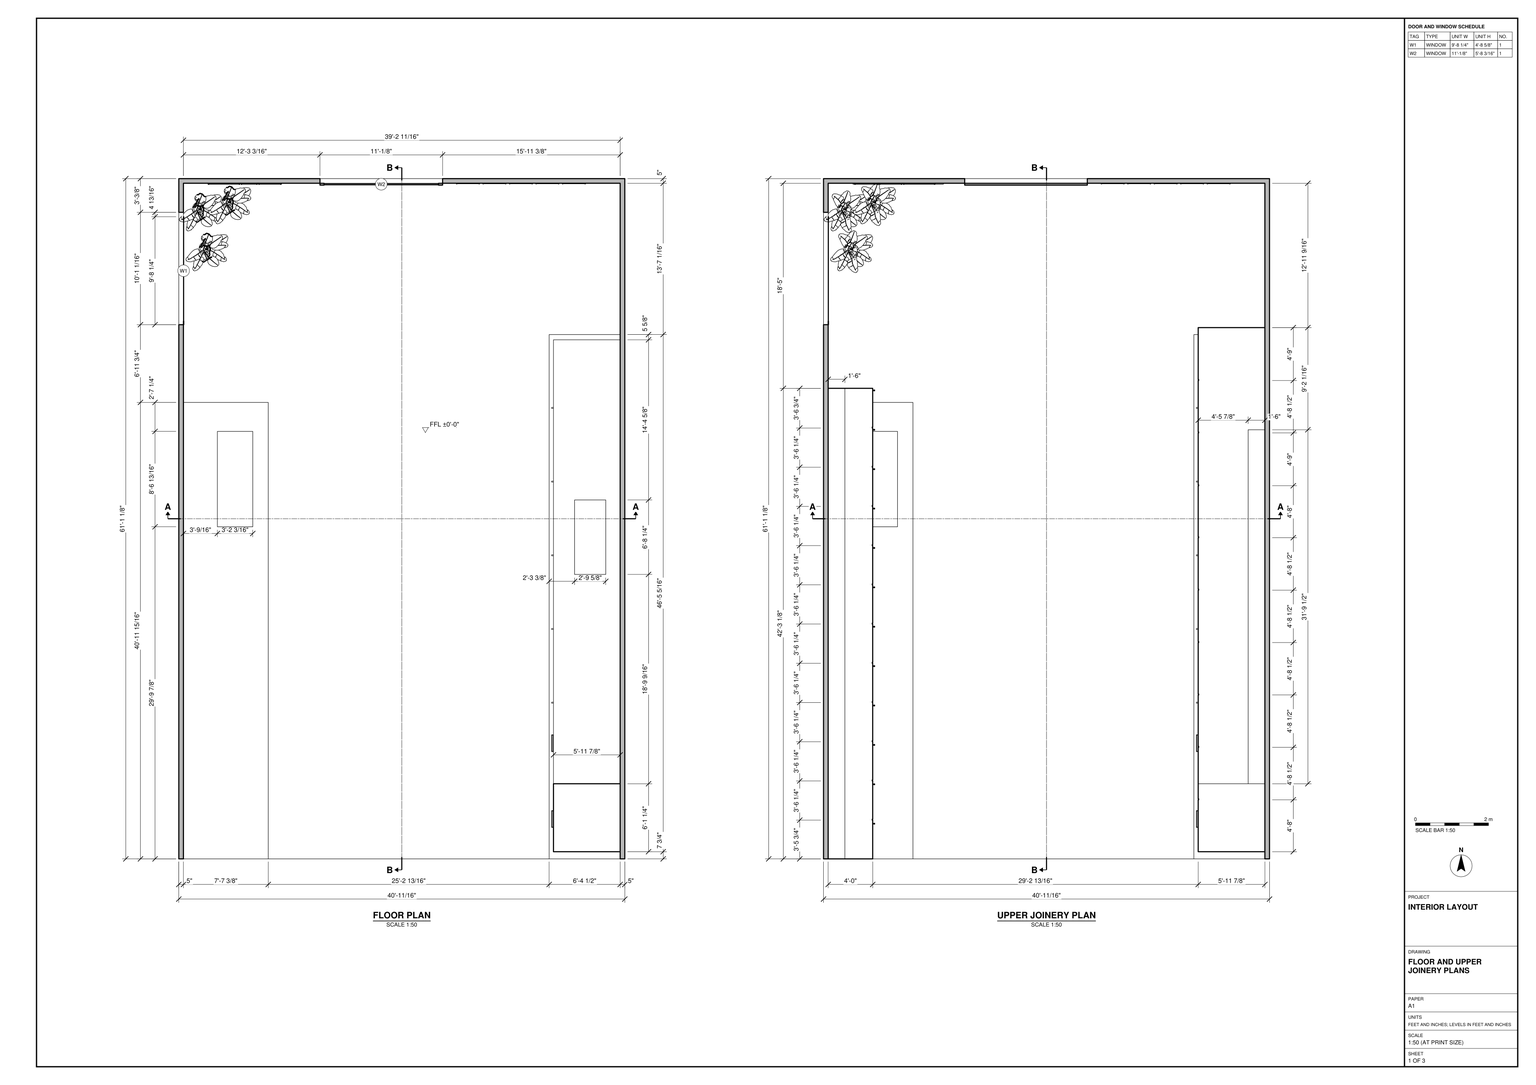
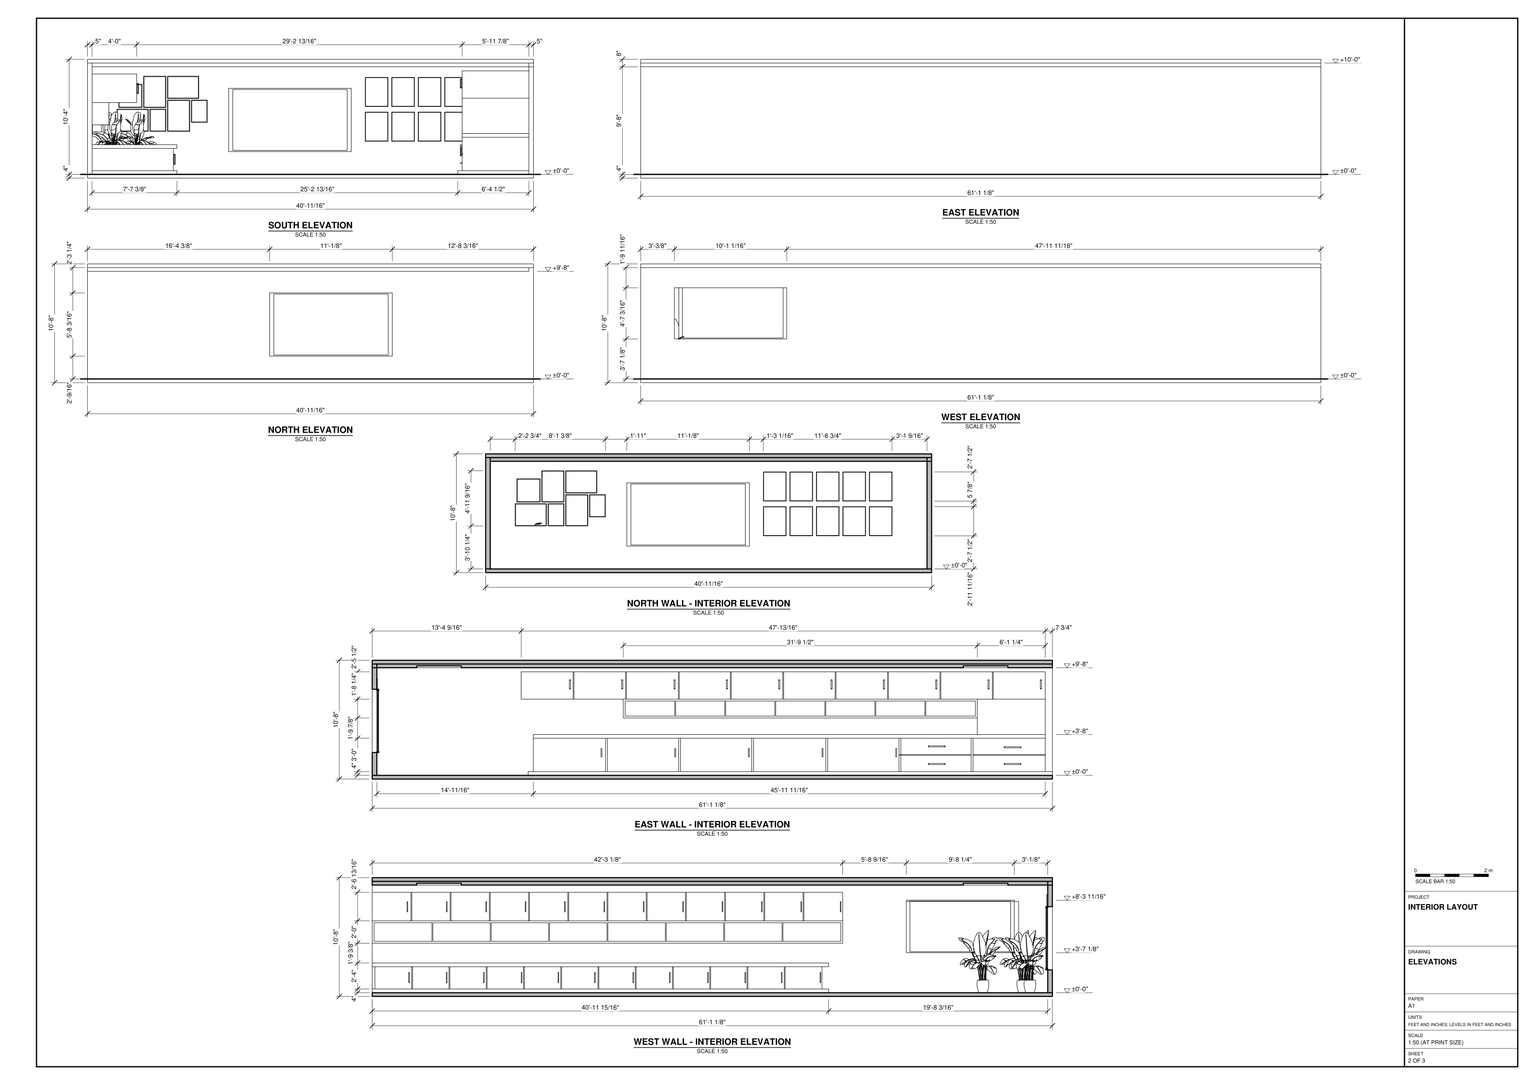
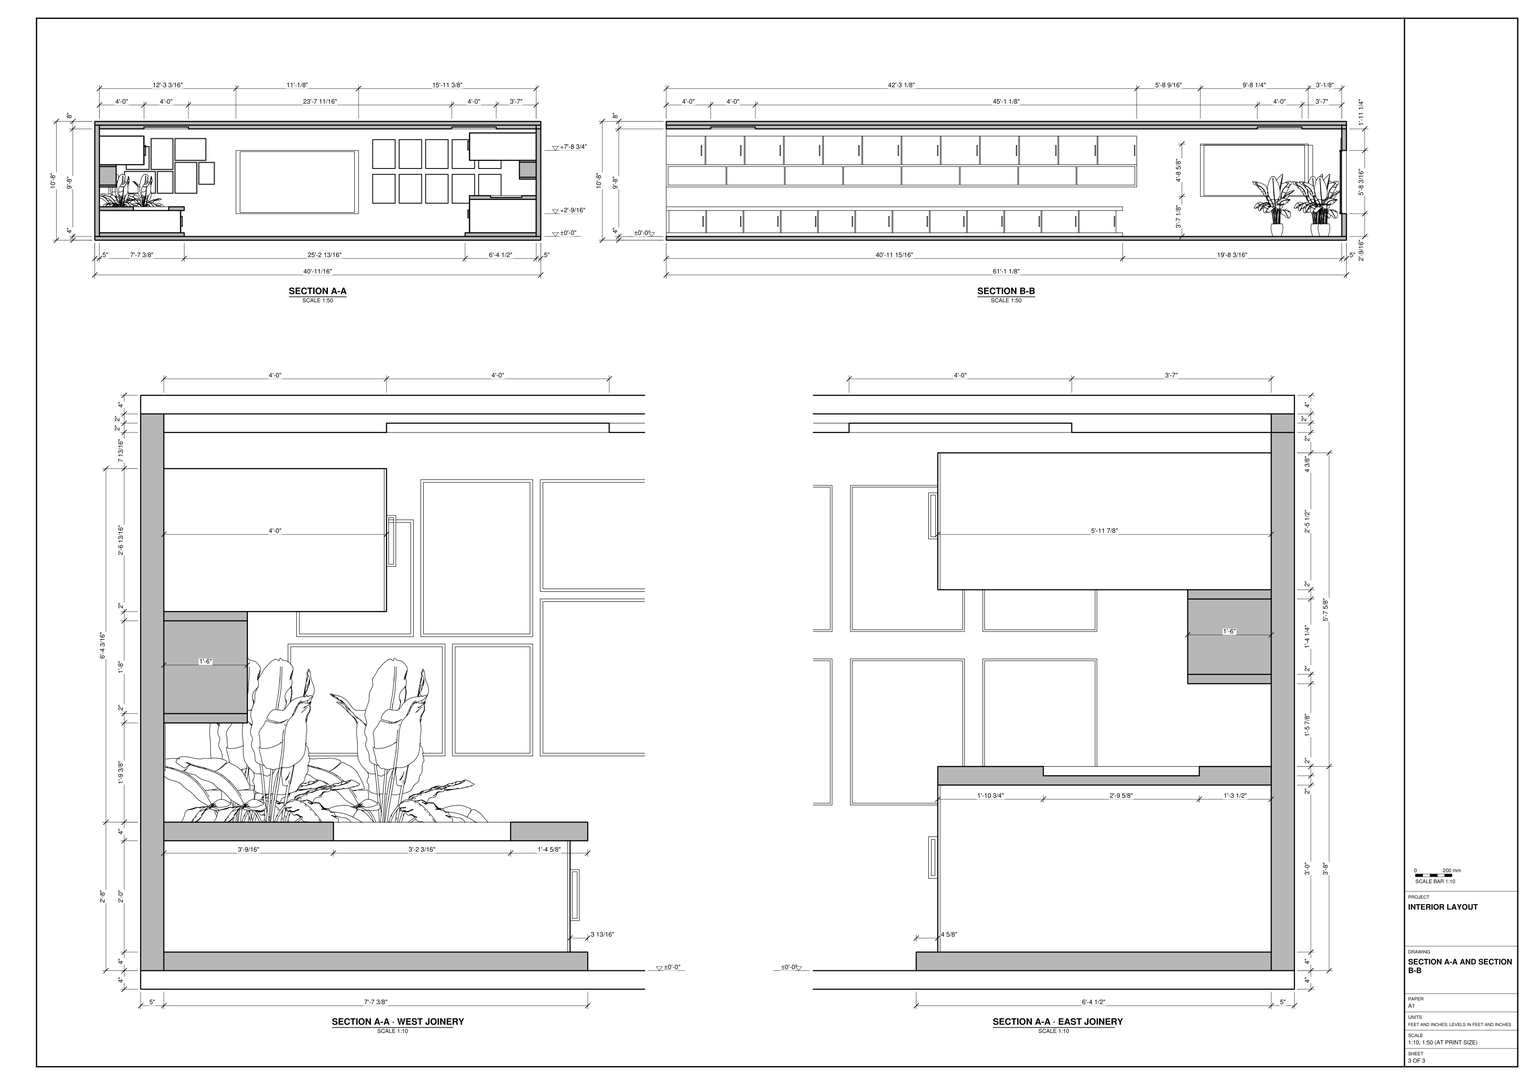
Build the interior shown in task_files/diagram_01.pdf in SketchUp. Work in feet and inches. Set the finished floor level to ±0'-0". The overall model is 40'-11/16" wide from west to east, 61'-1 1/8" long from south to north and 10'-8" high. Model the floor slab, the 5" walls on the west, north and east sides, and the flat overhead slab with the stepped underside shown in section. Leave the south end open. Fit one window in the north wall and the other near the north end of the west wall, using the plans and elevations to locate their jambs, heads and sills.

Build the two cabinet runs from the south end, leaving the central floor area clear. Use the floor plan for the base footprints and countertop recesses, and the upper joinery plan for the depths and limits of the wall cabinets. The west base is deeper and lower than the east base. Follow the enlarged sections for the plinths, cabinet fronts, countertop edges and shallow shelves beneath the upper cabinets. Match the door divisions, pulls and east-side drawers to the interior elevations. Place the plants near the northwest corner and the wall displays on either side of the north window. Decor and loose items may be any suitable library components.

Keep the walls, slabs and each joinery or furniture piece in separate groups or components, and use components for repeated parts. Save one SketchUp model as output_files/room_with_opposing_built_in_cabinet_runs.skp.

# SketchUp Ruby script. Lengths in inches.
U = 1.inch
M = Sketchup.active_model
def pt(a) = Geom::Point3d.new(a.map { |v| v * U })
def face(e, loops, mat)
  f = e.add_face(loops[0].map { |a| pt(a) })
  loops[1..].each { |l| e.add_face(l.map { |a| pt(a) }).erase! }
  f.material = f.back_material = mat if mat
  f
end
# faces: each face lists its corners as indices into pts; further lists are holes
def faces(e, pts, list, mat = nil) = list.each { |f| face(e, (f[0].is_a?(Array) ? f : [f]).map { |l| l.map { |i| pts[i] } }, mat) }
# xy, xz, yz: faces in a plane at the given z, y or x. An outline is a flat list of corners, or four numbers for a rectangle; further outlines are holes
def ring(l) = l.size == 4 ? [[l[0], l[1]], [l[2], l[1]], [l[2], l[3]], [l[0], l[3]]] : l.each_slice(2).to_a
def flat(e, list, mat, &to3) = list.each { |f| face(e, (f[0].is_a?(Array) ? f : [f]).map { |l| ring(l).map { |u, v| to3.(u, v) } }, mat) }
def xy(e, z, list, mat = nil) = flat(e, list, mat) { |x, y| [x, y, z] }
def xz(e, y, list, mat = nil) = flat(e, list, mat) { |x, z| [x, y, z] }
def yz(e, x, list, mat = nil) = flat(e, list, mat) { |y, z| [x, y, z] }
def lines(e, pts, list) = list.each { |a, b| e.add_line(pt(pts[a]), pt(pts[b])) }
# prism: a flat outline (further loops are holes) pulled along v
def prism(e, loops, v, mat = nil)
  f = face(e, loops, mat); d = Geom::Vector3d.new(v.map { |x| x * U })
  f.pushpull(f.normal.samedirection?(d) ? d.length : -d.length)
end
def box(e, o, s, mat = nil) = prism(e, [[o, [o[0] + s[0], o[1], o[2]], [o[0] + s[0], o[1] + s[1], o[2]], [o[0], o[1] + s[1], o[2]]]], [0, 0, s[2]], mat)
def at(x, y, z, deg = 0) = Geom::Transformation.translation(pt([x, y, z])) * Geom::Transformation.rotation(ORIGIN, Z_AXIS, deg.degrees)
def axes(o, x, y, z) = Geom::Transformation.new([*x, 0, *y, 0, *z, 0, *pt(o).to_a, 1])
def part(name) = M.definitions.add(name)
# library, detail: a bought-in or finely detailed component or shape, given as its bounding box
def library(name, o, s) = part(name).tap { |d| box(d.entities, o, s) }
def detail(e, o, s) = box(e.add_group.entities, o, s)
def put(e, d, t, mat = nil) = e.add_instance(d, t).tap { |i| i.material = mat if mat }
def group(e, t, mat = nil) = e.add_group.tap { |g| g.transformation = t; g.material = mat if mat }.entities
root = M.entities
M.materials.add("Emissive").color = [255, 255, 255]
M.materials.add("Mulheres-6-site1").color = [244, 244, 244]
M.materials.add("VOA-01-site1").color = [234, 234, 234]
M.materials.add("[Color E01]").color = [255, 255, 204]
M.materials.add("[Color F01]").color = [229, 255, 204]
M.materials.add("[Color F02]").color = [204, 255, 153]
M.materials.add("[Color M04]").color = [142, 142, 142]
M.materials.add("[Color M07]").color = [58, 58, 58]
M.materials.add("[Color_008]").color = [30, 30, 30]
M.materials.add("[Metal Seamed]").color = [118, 119, 115]
M.materials.add("[Slate Light Tile]1").color = [54, 54, 54]
M.materials.add("[Stone Brushed Khaki]").color = [226, 197, 133]
M.materials.add("[Translucent Glass Gray]3").color = [128, 128, 128]
M.materials["[Translucent Glass Gray]3"].alpha = 0.3
M.materials.add("[Translucent Glass Sky Reflection]").color = [126, 138, 183]
M.materials["[Translucent Glass Sky Reflection]"].alpha = 0.52
M.materials.add("[Wood Floor]").color = [117, 79, 46]
M.materials.add("despertar").color = [181, 181, 181]
M.materials.add("folhas").color = [175, 175, 175]
M.materials.add("nature-line").color = [164, 163, 166]
M.materials.add("wing").color = [211, 211, 211]
M.materials.add("woods 2").color = [211, 213, 213]
c1 = part("WINDOW (1)")
xy(c1.entities,0,[[0,0,59.06,1.97]],"[Color M07]")
xy(c1.entities,1.97,[[1.97,0,57.09,0.98],[1.97,0.98,57.09,1.97]],"[Color M07]")
xy(c1.entities,104.33,[[1.97,0,57.09,0.98],[1.97,0.98,57.09,1.97]],"[Color M07]")
xy(c1.entities,106.3,[[0,0,59.06,1.97]],"[Color M07]")
xz(c1.entities,0,[[[0,0,59.06,106.3],[1.97,1.97,57.09,104.33]]],"[Color M07]")
xz(c1.entities,0.98,[[1.97,1.97,57.09,104.33]],"[Translucent Glass Gray]3")
xz(c1.entities,1.97,[[[0,0,59.06,106.3],[1.97,1.97,57.09,104.33]]],"[Color M07]")
yz(c1.entities,0,[[0,0,1.97,106.3]],"[Color M07]")
yz(c1.entities,1.97,[[0,1.97,0.98,104.33],[0.98,1.97,1.97,104.33]],"[Color M07]")
yz(c1.entities,57.09,[[0,1.97,0.98,104.33],[0.98,1.97,1.97,104.33]],"[Color M07]")
yz(c1.entities,59.06,[[0,0,1.97,106.3]],"[Color M07]")
c2 = library("Baneira",[-21.22,-27.99,0],[51.24,48.13,67.625])
c3 = part("Cabinet panel")
xy(c3.entities,0,[[[0,0,24.61,31.5],[0.39,0.39,24.21,31.1]]],"[Color_008]")
xy(c3.entities,0.2,[[0.39,0.39,24.21,31.1]],"[Color_008]")
xy(c3.entities,0.59,[[[0,0,24.61,31.5],[0.39,0.39,24.21,31.1]]],"[Color_008]")
xz(c3.entities,0,[[0,0,24.61,0.59]],"[Color_008]")
xz(c3.entities,0.39,[[0.39,0.2,24.21,0.59]],"[Color_008]")
xz(c3.entities,31.1,[[0.39,0.2,24.21,0.59]],"[Color_008]")
xz(c3.entities,31.5,[[0,0,24.61,0.59]],"[Color_008]")
yz(c3.entities,0,[[0,0,31.5,0.59]],"[Color_008]")
yz(c3.entities,0.39,[[0.39,0.2,31.1,0.59]],"[Color_008]")
yz(c3.entities,24.21,[[0.39,0.2,31.1,0.59]],"[Color_008]")
yz(c3.entities,24.61,[[0,0,31.5,0.59]],"[Color_008]")
c4 = part("black+and+white+pictures")
g1 = group(c4.entities,at(0,0.875,14.87))
g2 = group(g1,at(0,0,0))
put(g2,c3,axes([0,0,0],[1,0,0],[0,0,1],[0,-1,0]))
g3 = group(g1,at(57.09,0,37.4))
put(g3,c3,axes([0,0,0],[1,0,0],[0,0,1],[0,-1,0]))
g4 = group(g1,at(28.54,0,37.4))
put(g4,c3,axes([0,0,0],[1,0,0],[0,0,1],[0,-1,0]))
g5 = group(g1,at(0,0,37.4))
put(g5,c3,axes([0,0,0],[1,0,0],[0,0,1],[0,-1,0]))
g6 = group(g1,at(114.17,0,0))
put(g6,c3,axes([0,0,0],[1,0,0],[0,0,1],[0,-1,0]))
g7 = group(g1,at(85.63,0,0))
put(g7,c3,axes([0,0,0],[1,0,0],[0,0,1],[0,-1,0]))
g8 = group(g1,at(57.09,0,0))
put(g8,c3,axes([0,0,0],[1,0,0],[0,0,1],[0,-1,0]))
g9 = group(g1,at(28.54,0,0))
put(g9,c3,axes([0,0,0],[1,0,0],[0,0,1],[0,-1,0]))
g10 = group(g1,at(114.17,0,37.4))
put(g10,c3,axes([0,0,0],[1,0,0],[0,0,1],[0,-1,0]))
g11 = group(g1,at(85.63,0,37.4))
put(g11,c3,axes([0,0,0],[1,0,0],[0,0,1],[0,-1,0]))
c5 = part("Agrupar\#3")
xy(c5.entities,0,[[0,0,24.13,1.1]])
xy(c5.entities,0.59,[[0.59,0,23.54,0.39]])
xy(c5.entities,33.27,[[0.59,0,23.54,0.39]])
xy(c5.entities,33.86,[[0,0,24.13,1.1]])
xz(c5.entities,0,[[[0,0,24.13,33.86],[0.59,0.59,23.54,33.27]]])
xz(c5.entities,0.39,[[0.59,0.59,23.54,33.27]],"nature-line")
xz(c5.entities,1.1,[[0,0,24.13,33.86]])
yz(c5.entities,0,[[0,0,1.1,33.86]])
yz(c5.entities,0.59,[[0,0.59,0.39,33.27]])
yz(c5.entities,23.54,[[0,0.59,0.39,33.27]])
yz(c5.entities,24.13,[[0,0,1.1,33.86]])
c6 = part("Agrupar\#1")
xy(c6.entities,0,[[0,0,24.13,1.1]])
xy(c6.entities,0.59,[[0.59,0,23.54,0.39]])
xy(c6.entities,33.27,[[0.59,0,23.54,0.39]])
xy(c6.entities,33.86,[[0,0,24.13,1.1]])
xz(c6.entities,0,[[[0,0,24.13,33.86],[0.59,0.59,23.54,33.27]]])
xz(c6.entities,0.39,[[0.59,0.59,23.54,33.27]],"despertar")
xz(c6.entities,1.1,[[0,0,24.13,33.86]])
yz(c6.entities,0,[[0,0,1.1,33.86]])
yz(c6.entities,0.59,[[0,0.59,0.39,33.27]])
yz(c6.entities,23.54,[[0,0.59,0.39,33.27]])
yz(c6.entities,24.13,[[0,0,1.1,33.86]])
c7 = part("Agrupar\#4")
xy(c7.entities,0,[[0,0,17.32,1.1]])
xy(c7.entities,0.59,[[0.59,0,16.73,0.39]])
xy(c7.entities,23.54,[[0.59,0,16.73,0.39]])
xy(c7.entities,24.13,[[0,0,17.32,1.1]])
xz(c7.entities,0,[[[0,0,17.32,24.13],[0.59,0.59,16.73,23.54]]])
xz(c7.entities,0.39,[[0.59,0.59,16.73,23.54]],"Mulheres-6-site1")
xz(c7.entities,1.1,[[0,0,17.32,24.13]])
yz(c7.entities,0,[[0,0,1.1,24.13]])
yz(c7.entities,0.59,[[0,0.59,0.39,23.54]])
yz(c7.entities,16.73,[[0,0.59,0.39,23.54]])
yz(c7.entities,17.32,[[0,0,1.1,24.13]])
c8 = part("Agrupar\#6")
xy(c8.entities,0,[[0,0,24.13,1.1]])
xy(c8.entities,0.59,[[0.59,0,23.54,0.39]])
xy(c8.entities,33.27,[[0.59,0,23.54,0.39]])
xy(c8.entities,33.86,[[0,0,24.13,1.1]])
xz(c8.entities,0,[[[0,0,24.13,33.86],[0.59,0.59,23.54,33.27]]])
xz(c8.entities,0.39,[[0.59,0.59,23.54,33.27]],"wing")
xz(c8.entities,1.1,[[0,0,24.13,33.86]])
yz(c8.entities,0,[[0,0,1.1,33.86]])
yz(c8.entities,0.59,[[0,0.59,0.39,33.27]])
yz(c8.entities,23.54,[[0,0.59,0.39,33.27]])
yz(c8.entities,24.13,[[0,0,1.1,33.86]])
c9 = part("Agrupar\#2")
xy(c9.entities,0,[[0,0,17.32,1.1]])
xy(c9.entities,0.59,[[0.59,0,16.73,0.39]])
xy(c9.entities,23.54,[[0.59,0,16.73,0.39]])
xy(c9.entities,24.13,[[0,0,17.32,1.1]])
xz(c9.entities,0,[[[0,0,17.32,24.13],[0.59,0.59,16.73,23.54]]])
xz(c9.entities,0.39,[[0.59,0.59,16.73,23.54]],"folhas")
xz(c9.entities,1.1,[[0,0,17.32,24.13]])
yz(c9.entities,0,[[0,0,1.1,24.13]])
yz(c9.entities,0.59,[[0,0.59,0.39,23.54]])
yz(c9.entities,16.73,[[0,0.59,0.39,23.54]])
yz(c9.entities,17.32,[[0,0,1.1,24.13]])
c10 = part("Agrupar\#5")
xy(c10.entities,0,[[0,0,24.13,1.1]])
xy(c10.entities,0.59,[[0.59,0,23.54,0.39]])
xy(c10.entities,33.27,[[0.59,0,23.54,0.39]])
xy(c10.entities,33.86,[[0,0,24.13,1.1]])
xz(c10.entities,0,[[[0,0,24.13,33.86],[0.59,0.59,23.54,33.27]]])
xz(c10.entities,0.39,[[0.59,0.59,23.54,33.27]],"VOA-01-site1")
xz(c10.entities,1.1,[[0,0,24.13,33.86]])
yz(c10.entities,0,[[0,0,1.1,33.86]])
yz(c10.entities,0.59,[[0,0.59,0.39,33.27]])
yz(c10.entities,23.54,[[0,0.59,0.39,33.27]])
yz(c10.entities,24.13,[[0,0,1.1,33.86]])
c11 = part("Agrupar\#19")
xy(c11.entities,0,[[0,0,25.2,1.1]],"[Color_008]")
xy(c11.entities,0.59,[[0.59,0,24.61,0.39]],"[Color_008]")
xy(c11.entities,24.61,[[0.59,0,24.61,0.39]],"[Color_008]")
xy(c11.entities,25.2,[[0,0,25.2,1.1]],"[Color_008]")
xz(c11.entities,0,[[[0,0,25.2,25.2],[0.59,0.59,24.61,24.61]]],"[Color_008]")
xz(c11.entities,0.39,[[0.59,0.59,24.61,24.61]],"woods 2")
xz(c11.entities,1.1,[[0,0,25.2,25.2]],"[Color_008]")
yz(c11.entities,0,[[0,0,1.1,25.2]],"[Color_008]")
yz(c11.entities,0.59,[[0,0.59,0.39,24.61]],"[Color_008]")
yz(c11.entities,24.61,[[0,0.59,0.39,24.61]],"[Color_008]")
yz(c11.entities,25.2,[[0,0,1.1,25.2]],"[Color_008]")
c12 = part("Composicao+7+-+A1+A2+62")
put(c12.entities,c5,at(294.8,0,58.93),"[Color_008]")
put(c12.entities,c6,at(320.54,0,33.22),"[Color_008]")
put(c12.entities,c7,at(301.62,0,33.22),"[Color_008]")
put(c12.entities,c8,axes([266.18,0,57.36],[0,0,-1],[0,1,0],[1,0,0]),"[Color_008]")
put(c12.entities,c9,at(346.25,0,42.95),"[Color_008]")
put(c12.entities,c10,axes([354.4,0,68.66],[0,0,1],[0,1,0],[-1,0,0]),"[Color_008]")
put(c12.entities,c11,at(268.03,0,58.93),"[Color_008]")
c13 = part("Group\#13")
prism(c13.entities,[[[0,0.74,0],[0,0.74,10.99],[2,0.74,10.99],[2,0.74,0]],[[0.46,0.74,0.46],[1.54,0.74,0.46],[1.54,0.74,10.53],[0.46,0.74,10.53]]],[0,-0.74,0])
c14 = part("Group\#14")
xy(c14.entities,0,[[0,0,2,1.25]],"[Metal Seamed]")
xy(c14.entities,0.49,[[0.49,0,1.51,1.25]],"[Metal Seamed]")
xy(c14.entities,9.45,[[0.49,0,1.51,1.25]],"[Metal Seamed]")
xy(c14.entities,9.9375,[[0,0,2,1.25]],"[Metal Seamed]")
xz(c14.entities,0,[[[0,0,2,9.9375],[0.49,0.49,1.51,9.45]]],"[Metal Seamed]")
xz(c14.entities,1.25,[[[0,0,2,9.9375],[0.49,0.49,1.51,9.45]]],"[Metal Seamed]")
yz(c14.entities,0,[[0,0,1.25,9.9375]],"[Metal Seamed]")
yz(c14.entities,0.49,[[0,0.49,1.25,9.45]],"[Metal Seamed]")
yz(c14.entities,1.51,[[0,0.49,1.25,9.45]],"[Metal Seamed]")
yz(c14.entities,2,[[0,0,1.25,9.9375]])
c15 = part("Group\#15")
prism(c15.entities,[[[2,1.0625,9],[2,1.0625,0],[0,1.0625,0],[0,1.0625,9]],[[1.39,1.0625,0.61],[1.39,1.0625,8.39],[0.61,1.0625,8.39],[0.61,1.0625,0.61]]],[0,-1.0625,0])
c16 = part("Group\#16")
prism(c16.entities,[[[2,18.25,0],[2,0,0],[0,0,0],[0,18.25,0]],[[1.55,0.45,0],[1.55,17.8,0],[0.45,17.8,0],[0.45,0.45,0]]],[0,0,1.25])
xy(root,120,[[[5,0,480.6875,733.125],[53,48,432.6875,685.125]],[101,96,384.6875,637.125]],"[Color F01]")
xy(root,122,[[[53,48,432.6875,685.125],[101,96,384.6875,637.125]]],"[Color F01]")
xy(root,124,[[5,0,480.6875,733.125]])
xz(root,0,[[5,120,480.6875,124]])
xz(root,48,[[53,120,432.6875,122]])
xz(root,96,[[101,120,384.6875,122]],"Emissive")
xz(root,637.125,[[101,120,384.6875,122]])
xz(root,685.125,[[53,120,432.6875,122]])
xz(root,733.125,[[5,120,480.6875,124]])
yz(root,5,[[0,120,733.125,124]])
yz(root,23,[[2,59.4,64.39,79.4],[65.39,59.4,127.28,79.4],[128.28,59.4,190.17,79.4],[191.17,59.4,253.0625,79.4],[254.0625,59.4,315.95,79.4],
  [316.95,59.4,378.84,79.4],[379.84,59.4,441.73,79.4],[442.73,59.4,505.125,79.4]],"[Translucent Glass Sky Reflection]")
yz(root,53,[[48,120,685.125,122]])
yz(root,101,[[96,120,637.125,122]],"Emissive")
yz(root,384.6875,[[96,120,637.125,122]],"Emissive")
yz(root,432.6875,[[48,120,685.125,122]])
yz(root,457.6875,[[82.97,67.85,136.4,84.1],[137.4,67.85,190.33,84.1],[191.33,67.85,244.26,84.1],[245.26,67.85,298.1875,84.1],[299.1875,67.85,352.12,84.1],
  [353.12,67.85,406.05,84.1],[407.05,67.85,460.47,84.1]],"[Translucent Glass Sky Reflection]")
yz(root,480.6875,[[0,120,733.125,124]])
put(root,c1,axes([152.17,726.1,28.58],[2.23732,0,0],[0,1,0],[0,0,0.64147]))
put(root,c1,axes([5.31,575.7,47.12],[0,1.96884,0],[-0.16,0,0],[0,0,0.53242]))
put(root,c2,at(19.35,700.29,4))
put(root,c2,at(26.4,657.3,4))
put(root,c2,at(51.02,707.99,4))
put(root,c4,at(299.34,727.25,24.82))
put(root,c12,at(-234.42,727.02,17.05))
g12 = group(root,at(0,0,0),"[Stone Brushed Khaki]")
box(g12,[0,0,0],[480.6875,733.125,4])
g13 = group(root,at(0,0,4),"[Color E01]")
xy(g13,24.58,[[152.17,728.125,284.3,733.125]])
xy(g13,43.12,[[0,575.7,5,696.77]])
xy(g13,92.77,[[152.17,728.125,284.3,733.125]])
xy(g13,98.31,[[0,575.7,5,696.77]])
xy(g13,120,[[0,0,5,0,5,728.125,475.6875,728.125,475.6875,0,480.6875,0,480.6875,733.125,0,733.125]])
xz(g13,0,[[0,0,5,120],[475.6875,0,480.6875,120]])
xz(g13,575.7,[[0,43.12,5,98.31]])
xz(g13,696.77,[[0,43.12,5,98.31]])
xz(g13,728.125,[[[5,0,475.6875,120],[152.17,24.58,284.3,92.77]]])
xz(g13,733.125,[[[0,0,480.6875,120],[152.17,24.58,284.3,92.77]]])
yz(g13,0,[[[0,0,733.125,120],[575.7,43.12,696.77,98.31]]])
yz(g13,5,[[[0,0,728.125,120],[575.7,43.12,696.77,98.31]]])
yz(g13,152.17,[[728.125,24.58,733.125,92.77]])
yz(g13,284.3,[[728.125,24.58,733.125,92.77]])
yz(g13,475.6875,[[0,0,728.125,120]])
yz(g13,480.6875,[[0,0,733.125,120]])
p = [[5,0,0],[475.6875,0,0]]
lines(g13,p,[[0,1]])
g14 = group(root,at(0,0,124))
box(g14,[0,0,0],[480.6875,733.125,4])
g15 = group(root,at(399.17,0,4),"[Color F02]")
box(g15,[0,0,0],[76.52,565.05,4])
g16 = group(root,at(403.8125,7.72,8),"[Color F02]")
xy(g16,0,[[0,0,0,77.81,0.5,77.81,0.5,79.81,0,79.81,0,155.63,0.5,155.63,0.5,157.63,0,157.63,0,234.44,0.5,234.44,0.5,236.44,0,236.44,0,314.26,0.5,314.26,0.5,316.26,0,316.26,0,393.07,0.5,393.07,0.5,395.07,0,395.07,0,471.89,0.5,471.89,0.5,473.89,0,473.89,0,551.7,71.875,551.7,71.875,0]])
xy(g16,17.5,[[0,0,0.5,77.81],[0,79.81,0.5,155.63]])
xy(g16,18.5,[[0,0,0.5,77.81],[0,79.81,0.5,155.63]])
xy(g16,36,[[0,0,71.875,0,71.875,551.7,0,551.7,0,473.89,0.5,473.89,0.5,471.89,0,471.89,0,395.07,0.5,395.07,0.5,393.07,0,393.07,0,316.26,0.5,316.26,0.5,314.26,0,314.26,0,236.44,0.5,236.44,0.5,234.44,0,234.44,0,157.63,0.5,157.63,0.5,155.63,0,155.63,0,79.81,0.5,79.81,0.5,77.81,0,77.81]])
xz(g16,0,[[0,0,71.875,0,71.875,36,0,36,0,18.5,0.5,18.5,0.5,17.5,0,17.5]])
xz(g16,77.81,[[0,0,0.5,17.5],[0,18.5,0.5,36]])
xz(g16,79.81,[[0,0,0.5,17.5],[0,18.5,0.5,36]])
xz(g16,155.63,[[0,0,0.5,17.5],[0,18.5,0.5,36]])
xz(g16,157.63,[[0,0,0.5,17.5],[0,17.5,0.5,18.5],[0,18.5,0.5,36]])
xz(g16,234.44,[[0,0,0.5,36]])
xz(g16,236.44,[[0,0,0.5,36]])
xz(g16,314.26,[[0,0,0.5,36]])
xz(g16,316.26,[[0,0,0.5,36]])
xz(g16,393.07,[[0,0,0.5,36]])
xz(g16,395.07,[[0,0,0.5,36]])
xz(g16,471.89,[[0,0,0.5,36]])
xz(g16,473.89,[[0,0,0.5,36]])
xz(g16,551.7,[[0,0,71.875,36]])
yz(g16,0,[[0,0,77.81,17.5],[79.81,0,155.63,17.5],[157.63,0,234.44,36],[236.44,0,314.26,36],[316.26,0,393.07,36],
  [395.07,0,471.89,36],[473.89,0,551.7,36],[0,18.5,77.81,36],[79.81,18.5,155.63,36]])
yz(g16,0.5,[[77.81,0,79.81,36],[155.63,0,157.63,17.5],[234.44,0,236.44,36],[314.26,0,316.26,36],[393.07,0,395.07,36],
  [471.89,0,473.89,36],[0,17.5,77.81,18.5],[79.81,17.5,155.63,18.5],[155.63,17.5,157.63,18.5],[155.63,18.5,157.63,36]])
yz(g16,71.875,[[0,0,551.7,36]])
g17 = group(root,at(399.17,0,44),"[Slate Light Tile]1")
xy(g17,0,[[4.65,7.72,76.52,559.43]])
xy(g17,2,[[27.39,306.56,61.02,386.81]])
xy(g17,4,[[[4.65,7.72,76.52,559.43],[27.39,306.56,61.02,386.81]]])
xz(g17,7.72,[[4.65,0,76.52,4]])
xz(g17,306.56,[[27.39,2,61.02,4]])
xz(g17,386.81,[[27.39,2,61.02,4]])
xz(g17,559.43,[[4.65,0,76.52,4]])
yz(g17,4.65,[[7.72,0,559.43,4]])
yz(g17,27.39,[[306.56,2,386.81,4]])
yz(g17,61.02,[[306.56,2,386.81,4]])
yz(g17,76.52,[[7.72,0,559.43,4]])
g18 = group(root,at(403.8125,0,86.1),"[Color E01]")
prism(g18,[[[71.875,572.5625,0],[71.875,7.72,0],[0,7.72,0],[0,63.71,0],[0.5,63.71,0],[0.5,64.71,0],[0,64.71,0],[0,120.19,0],[0.5,120.19,0],[0.5,121.19,0],[0,121.19,0],[0,176.68,0],[0.5,176.68,0],[0.5,177.68,0],[0,177.68,0],[0,233.16,0],[0.5,233.16,0],[0.5,234.16,0],[0,234.16,0],[0,289.64,0],[0.5,289.64,0],[0.5,290.64,0],[0,290.64,0],[0,346.13,0],[0.5,346.13,0],[0.5,347.13,0],[0,347.13,0],[0,402.11,0],[0.5,402.11,0],[0.5,403.11,0],[0,403.11,0],[0,459.09,0],[0.5,459.09,0],[0.5,460.09,0],[0,460.09,0],[0,515.58,0],[0.5,515.58,0],[0.5,516.58,0],[0,516.58,0],[0,572.5625,0]]],[0,0,29.5])
g19 = group(root,at(403.8125,7.72,48),"[Color M04]")
xy(g19,0,[[0,0,71.875,73.25]])
xy(g19,17.85,[[53.875,73.25,71.875,454.75]],"[Wood Floor]")
xy(g19,19.85,[[53.875,75.25,71.875,128.68],[53.875,129.68,71.875,182.61],[53.875,183.61,71.875,236.54],[53.875,237.54,71.875,290.46],[53.875,291.46,71.875,344.39],
  [53.875,345.39,71.875,398.32],[53.875,399.32,71.875,452.75]])
xy(g19,36.1,[[53.875,75.25,71.875,128.68],[53.875,129.68,71.875,182.61],[53.875,183.61,71.875,236.54],[53.875,237.54,71.875,290.46],[53.875,291.46,71.875,344.39],
  [53.875,345.39,71.875,398.32],[53.875,399.32,71.875,452.75]])
xy(g19,38.1,[[0,0,71.875,73.25],[53.875,73.25,71.875,454.75]])
xz(g19,0,[[0,0,71.875,38.1]])
xz(g19,73.25,[[0,0,0,38.1,53.875,38.1,53.875,17.85,71.875,17.85,71.875,0],[53.875,17.85,71.875,38.1]])
xz(g19,75.25,[[53.875,19.85,71.875,36.1]],"[Wood Floor]")
xz(g19,128.68,[[53.875,19.85,71.875,36.1]],"[Wood Floor]")
xz(g19,129.68,[[53.875,19.85,71.875,36.1]],"[Wood Floor]")
xz(g19,182.61,[[53.875,19.85,71.875,36.1]],"[Wood Floor]")
xz(g19,183.61,[[53.875,19.85,71.875,36.1]],"[Wood Floor]")
xz(g19,236.54,[[53.875,19.85,71.875,36.1]],"[Wood Floor]")
xz(g19,237.54,[[53.875,19.85,71.875,36.1]],"[Wood Floor]")
xz(g19,290.46,[[53.875,19.85,71.875,36.1]],"[Wood Floor]")
xz(g19,291.46,[[53.875,19.85,71.875,36.1]],"[Wood Floor]")
xz(g19,344.39,[[53.875,19.85,71.875,36.1]],"[Wood Floor]")
xz(g19,345.39,[[53.875,19.85,71.875,36.1]],"[Wood Floor]")
xz(g19,398.32,[[53.875,19.85,71.875,36.1]],"[Wood Floor]")
xz(g19,399.32,[[53.875,19.85,71.875,36.1]],"[Wood Floor]")
xz(g19,452.75,[[53.875,19.85,71.875,36.1]],"[Wood Floor]")
xz(g19,454.75,[[53.875,17.85,71.875,38.1]],"[Wood Floor]")
yz(g19,0,[[0,0,73.25,38.1]])
yz(g19,53.875,[[[73.25,17.85,454.75,38.1],[75.25,19.85,128.68,36.1],[399.32,19.85,452.75,36.1],[345.39,19.85,398.32,36.1],[237.54,19.85,290.46,36.1],[183.61,19.85,236.54,36.1],[129.68,19.85,182.61,36.1],[291.46,19.85,344.39,36.1]]],"[Wood Floor]")
yz(g19,71.875,[[0,0,73.25,38.1],[[73.25,17.85,454.75,38.1],[75.25,19.85,128.68,36.1],[399.32,19.85,452.75,36.1],[345.39,19.85,398.32,36.1],[237.54,19.85,290.46,36.1],[183.61,19.85,236.54,36.1],[129.68,19.85,182.61,36.1],[291.46,19.85,344.39,36.1]]])
yz(g19,71.875,[[75.25,19.85,128.68,36.1],[129.68,19.85,182.61,36.1],[183.61,19.85,236.54,36.1],[237.54,19.85,290.46,36.1],[291.46,19.85,344.39,36.1],
  [345.39,19.85,398.32,36.1],[399.32,19.85,452.75,36.1]],"[Wood Floor]")
g20 = group(root,at(5,0,4),"[Color F02]")
box(g20,[0,0,0],[91.375,491.9375,4])
g21 = group(root,at(5,9.19,8),"[Color F02]")
xy(g21,0,[[0,-6.25,0,475.5625,87.5625,475.5625,87.5625,435.91,87.0625,435.91,87.0625,434.91,87.5625,434.91,87.5625,395.76,87.0625,395.76,87.0625,394.76,87.5625,394.76,87.5625,355.61,87.0625,355.61,87.0625,354.61,87.5625,354.61,87.5625,315.46,87.0625,315.46,87.0625,314.46,87.5625,314.46,87.5625,275.31,87.0625,275.31,87.0625,274.31,87.5625,274.31,87.5625,235.16,87.0625,235.16,87.0625,234.16,87.5625,234.16,87.5625,195.01,87.0625,195.01,87.0625,194.01,87.5625,194.01,87.5625,154.85,87.0625,154.85,87.0625,153.85,87.5625,153.85,87.5625,114.7,87.0625,114.7,87.0625,113.7,87.5625,113.7,87.5625,74.55,87.0625,74.55,87.0625,73.55,87.5625,73.55,87.5625,34.4,87.0625,34.4,87.0625,33.4,87.5625,33.4,87.5625,-6.25]])
xy(g21,24,[[0,-6.25,87.5625,-6.25,87.5625,33.4,87.0625,33.4,87.0625,34.4,87.5625,34.4,87.5625,73.55,87.0625,73.55,87.0625,74.55,87.5625,74.55,87.5625,113.7,87.0625,113.7,87.0625,114.7,87.5625,114.7,87.5625,153.85,87.0625,153.85,87.0625,154.85,87.5625,154.85,87.5625,194.01,87.0625,194.01,87.0625,195.01,87.5625,195.01,87.5625,234.16,87.0625,234.16,87.0625,235.16,87.5625,235.16,87.5625,274.31,87.0625,274.31,87.0625,275.31,87.5625,275.31,87.5625,314.46,87.0625,314.46,87.0625,315.46,87.5625,315.46,87.5625,354.61,87.0625,354.61,87.0625,355.61,87.5625,355.61,87.5625,394.76,87.0625,394.76,87.0625,395.76,87.5625,395.76,87.5625,434.91,87.0625,434.91,87.0625,435.91,87.5625,435.91,87.5625,475.5625,0,475.5625]],"[Color E01]")
xy(g21,73.4,[[0,-9.19,0,497.93,48,497.93,48,456.17,47.5,456.17,47.5,455.17,48,455.17,48,413.91,47.5,413.91,47.5,412.91,48,412.91,48,371.65,47.5,371.65,47.5,370.65,48,370.65,48,329.39,47.5,329.39,47.5,328.39,48,328.39,48,287.13,47.5,287.13,47.5,286.13,48,286.13,48,244.87,47.5,244.87,47.5,243.87,48,243.87,48,202.61,47.5,202.61,47.5,201.61,48,201.61,48,160.35,47.5,160.35,47.5,159.35,48,159.35,48,118.09,47.5,118.09,47.5,117.09,48,117.09,48,75.83,47.5,75.83,47.5,74.83,48,74.83,48,33.57,47.5,33.57,47.5,32.57,48,32.57,48,-9.19]],"[Color E01]")
xy(g21,104.21,[[0,-9.19,48,-9.19,48,32.57,47.5,32.57,47.5,33.57,48,33.57,48,74.83,47.5,74.83,47.5,75.83,48,75.83,48,117.09,47.5,117.09,47.5,118.09,48,118.09,48,159.35,47.5,159.35,47.5,160.35,48,160.35,48,201.61,47.5,201.61,47.5,202.61,48,202.61,48,243.87,47.5,243.87,47.5,244.87,48,244.87,48,286.13,47.5,286.13,47.5,287.13,48,287.13,48,328.39,47.5,328.39,47.5,329.39,48,329.39,48,370.65,47.5,370.65,47.5,371.65,48,371.65,48,412.91,47.5,412.91,47.5,413.91,48,413.91,48,455.17,47.5,455.17,47.5,456.17,48,456.17,48,497.93,0,497.93]],"[Color E01]")
xz(g21,-9.19,[[0,73.4,48,104.21]],"[Color E01]")
xz(g21,-6.25,[[0,0,87.5625,24]])
xz(g21,32.57,[[47.5,73.4,48,104.21]])
xz(g21,33.4,[[87.0625,0,87.5625,24]])
xz(g21,33.57,[[47.5,73.4,48,104.21]])
xz(g21,34.4,[[87.0625,0,87.5625,24]])
xz(g21,73.55,[[87.0625,0,87.5625,24]])
xz(g21,74.55,[[87.0625,0,87.5625,24]])
xz(g21,74.83,[[47.5,73.4,48,104.21]])
xz(g21,75.83,[[47.5,73.4,48,104.21]])
xz(g21,113.7,[[87.0625,0,87.5625,24]])
xz(g21,114.7,[[87.0625,0,87.5625,24]])
xz(g21,117.09,[[47.5,73.4,48,104.21]])
xz(g21,118.09,[[47.5,73.4,48,104.21]])
xz(g21,153.85,[[87.0625,0,87.5625,24]])
xz(g21,154.85,[[87.0625,0,87.5625,24]])
xz(g21,159.35,[[47.5,73.4,48,104.21]])
xz(g21,160.35,[[47.5,73.4,48,104.21]])
xz(g21,194.01,[[87.0625,0,87.5625,24]])
xz(g21,195.01,[[87.0625,0,87.5625,24]])
xz(g21,201.61,[[47.5,73.4,48,104.21]])
xz(g21,202.61,[[47.5,73.4,48,104.21]])
xz(g21,234.16,[[87.0625,0,87.5625,24]])
xz(g21,235.16,[[87.0625,0,87.5625,24]])
xz(g21,243.87,[[47.5,73.4,48,104.21]])
xz(g21,244.87,[[47.5,73.4,48,104.21]])
xz(g21,274.31,[[87.0625,0,87.5625,24]])
xz(g21,275.31,[[87.0625,0,87.5625,24]])
xz(g21,286.13,[[47.5,73.4,48,104.21]])
xz(g21,287.13,[[47.5,73.4,48,104.21]])
xz(g21,314.46,[[87.0625,0,87.5625,24]])
xz(g21,315.46,[[87.0625,0,87.5625,24]])
xz(g21,328.39,[[47.5,73.4,48,104.21]])
xz(g21,329.39,[[47.5,73.4,48,104.21]])
xz(g21,354.61,[[87.0625,0,87.5625,24]])
xz(g21,355.61,[[87.0625,0,87.5625,24]])
xz(g21,370.65,[[47.5,73.4,48,104.21]])
xz(g21,371.65,[[47.5,73.4,48,104.21]])
xz(g21,394.76,[[87.0625,0,87.5625,24]])
xz(g21,395.76,[[87.0625,0,87.5625,24]])
xz(g21,412.91,[[47.5,73.4,48,104.21]])
xz(g21,413.91,[[47.5,73.4,48,104.21]])
xz(g21,434.91,[[87.0625,0,87.5625,24]])
xz(g21,435.91,[[87.0625,0,87.5625,24]])
xz(g21,455.17,[[47.5,73.4,48,104.21]])
xz(g21,456.17,[[47.5,73.4,48,104.21]])
xz(g21,475.5625,[[0,0,87.5625,24]])
xz(g21,497.93,[[0,73.4,48,104.21]],"[Color E01]")
yz(g21,0,[[-6.25,0,475.5625,24],[-9.19,73.4,497.93,104.21]])
yz(g21,47.5,[[32.57,73.4,33.57,104.21],[74.83,73.4,75.83,104.21],[117.09,73.4,118.09,104.21],[159.35,73.4,160.35,104.21],[201.61,73.4,202.61,104.21],
  [243.87,73.4,244.87,104.21],[286.13,73.4,287.13,104.21],[328.39,73.4,329.39,104.21],[370.65,73.4,371.65,104.21],[412.91,73.4,413.91,104.21],
  [455.17,73.4,456.17,104.21]],"[Color E01]")
yz(g21,48,[[-9.19,73.4,32.57,104.21],[33.57,73.4,74.83,104.21],[75.83,73.4,117.09,104.21],[118.09,73.4,159.35,104.21],[160.35,73.4,201.61,104.21],
  [202.61,73.4,243.87,104.21],[244.87,73.4,286.13,104.21],[287.13,73.4,328.39,104.21],[329.39,73.4,370.65,104.21],[371.65,73.4,412.91,104.21],
  [413.91,73.4,455.17,104.21],[456.17,73.4,497.93,104.21]],"[Color E01]")
yz(g21,87.0625,[[33.4,0,34.4,24],[73.55,0,74.55,24],[113.7,0,114.7,24],[153.85,0,154.85,24],[194.01,0,195.01,24],
  [234.16,0,235.16,24],[274.31,0,275.31,24],[314.46,0,315.46,24],[354.61,0,355.61,24],[394.76,0,395.76,24],
  [434.91,0,435.91,24]])
yz(g21,87.5625,[[-6.25,0,33.4,24],[34.4,0,73.55,24],[74.55,0,113.7,24],[114.7,0,153.85,24],[154.85,0,194.01,24],
  [195.01,0,234.16,24],[235.16,0,274.31,24],[275.31,0,314.46,24],[315.46,0,354.61,24],[355.61,0,394.76,24],
  [395.76,0,434.91,24],[435.91,0,475.5625,24]])
g22 = group(root,at(5,0,32),"[Slate Light Tile]1")
prism(g22,[[[0,491.9375,0],[91.375,491.9375,0],[91.375,0,0],[0,0,0]],[[74.74,357.89,0],[74.74,460.7,0],[36.56,460.7,0],[36.56,357.89,0]]],[0,0,4])
g23 = group(root,at(5,0,57.4),"[Wood Floor]")
xy(g23,0,[[0,0,18,507.125]])
xy(g23,2,[[0,2,18,64.39],[0,65.39,18,127.28],[0,128.28,18,190.17],[0,191.17,18,253.0625],[0,254.0625,18,315.95],
  [0,316.95,18,378.84],[0,379.84,18,441.73],[0,442.73,18,505.125]])
xy(g23,22,[[0,2,18,64.39],[0,65.39,18,127.28],[0,128.28,18,190.17],[0,191.17,18,253.0625],[0,254.0625,18,315.95],
  [0,316.95,18,378.84],[0,379.84,18,441.73],[0,442.73,18,505.125]])
xy(g23,24,[[0,0,18,507.125]])
xz(g23,0,[[0,0,18,24]])
xz(g23,2,[[0,2,18,22]])
xz(g23,64.39,[[0,2,18,22]])
xz(g23,65.39,[[0,2,18,22]])
xz(g23,127.28,[[0,2,18,22]])
xz(g23,128.28,[[0,2,18,22]])
xz(g23,190.17,[[0,2,18,22]])
xz(g23,191.17,[[0,2,18,22]])
xz(g23,253.0625,[[0,2,18,22]])
xz(g23,254.0625,[[0,2,18,22]])
xz(g23,315.95,[[0,2,18,22]])
xz(g23,316.95,[[0,2,18,22]])
xz(g23,378.84,[[0,2,18,22]])
xz(g23,379.84,[[0,2,18,22]])
xz(g23,441.73,[[0,2,18,22]])
xz(g23,442.73,[[0,2,18,22]])
xz(g23,505.125,[[0,2,18,22]])
xz(g23,507.125,[[0,0,18,24]])
yz(g23,0,[[[0,0,507.125,24],[2,2,64.39,22],[442.73,2,505.125,22],[379.84,2,441.73,22],[316.95,2,378.84,22],[254.0625,2,315.95,22],[191.17,2,253.0625,22],[128.28,2,190.17,22],[65.39,2,127.28,22]],[2,2,64.39,22],[65.39,2,127.28,22],[128.28,2,190.17,22],[191.17,2,253.0625,22],
  [254.0625,2,315.95,22],[316.95,2,378.84,22],[379.84,2,441.73,22],[442.73,2,505.125,22]])
yz(g23,18,[[[0,0,507.125,24],[2,2,64.39,22],[442.73,2,505.125,22],[379.84,2,441.73,22],[316.95,2,378.84,22],[254.0625,2,315.95,22],[191.17,2,253.0625,22],[128.28,2,190.17,22],[65.39,2,127.28,22]]])
put(root,c13,at(53,37.57,91.11),"[Metal Seamed]")
put(root,c13,at(53,80.02,91.11),"[Metal Seamed]")
put(root,c13,at(53,122.46,91.11),"[Metal Seamed]")
put(root,c13,at(53,164.91,91.11),"[Metal Seamed]")
put(root,c13,at(53,207.36,91.11),"[Metal Seamed]")
put(root,c13,at(53,249.8125,91.11),"[Metal Seamed]")
put(root,c13,at(53,292.26,91.11),"[Metal Seamed]")
put(root,c13,at(53,334.71,91.11),"[Metal Seamed]")
put(root,c13,at(53,377.16,91.11),"[Metal Seamed]")
put(root,c13,at(53,419.61,91.11),"[Metal Seamed]")
put(root,c13,at(53,462.06,91.11),"[Metal Seamed]")
put(root,c13,at(53,504.5,91.11),"[Metal Seamed]")
put(root,c13,at(92.5625,39.3,14.79),"[Metal Seamed]")
put(root,c13,at(92.5625,79.92,14.79),"[Metal Seamed]")
put(root,c13,at(92.5625,119.99,14.79),"[Metal Seamed]")
put(root,c13,at(92.5625,160.67,14.79),"[Metal Seamed]")
put(root,c13,at(92.5625,200.3,14.79),"[Metal Seamed]")
put(root,c13,at(92.5625,239.67,14.79),"[Metal Seamed]")
put(root,c13,at(92.5625,280.99,14.79),"[Metal Seamed]")
put(root,c13,at(92.5625,320.42,14.79),"[Metal Seamed]")
put(root,c13,at(92.5625,361.55,14.79),"[Metal Seamed]")
put(root,c13,at(92.5625,401.74,14.79),"[Metal Seamed]")
put(root,c13,at(92.5625,441.05,14.79),"[Metal Seamed]")
put(root,c13,at(92.5625,482.74,14.79),"[Metal Seamed]")
put(root,c14,at(401.8125,519.39,97.06))
put(root,c14,at(401.8125,462.99,97.06))
put(root,c14,at(401.8125,406.58,97.06))
put(root,c14,at(401.8125,350.18,97.06))
put(root,c14,at(401.8125,293.78,97.06))
put(root,c14,at(401.8125,237.375,97.06))
put(root,c14,at(401.8125,180.97,97.06))
put(root,c14,at(401.8125,124.57,97.06))
put(root,c14,at(401.8125,68.17,97.06))
put(root,c14,at(401.8125,11.77,97.06))
put(root,c15,at(401.8125,167.79,23.88),"[Metal Seamed]")
put(root,c15,at(401.8125,247.21,23.88),"[Metal Seamed]")
put(root,c15,at(401.8125,326.64,23.88),"[Metal Seamed]")
put(root,c15,at(401.8125,406.06,23.88),"[Metal Seamed]")
put(root,c15,at(401.8125,485.48,23.88),"[Metal Seamed]")
put(root,c16,at(401.8125,115.53,34.59),"[Metal Seamed]")
put(root,c16,at(401.8125,115.53,15.59),"[Metal Seamed]")
put(root,c16,at(401.8125,33.85,15.59),"[Metal Seamed]")
put(root,c16,at(401.8125,33.85,33.65),"[Metal Seamed]")
